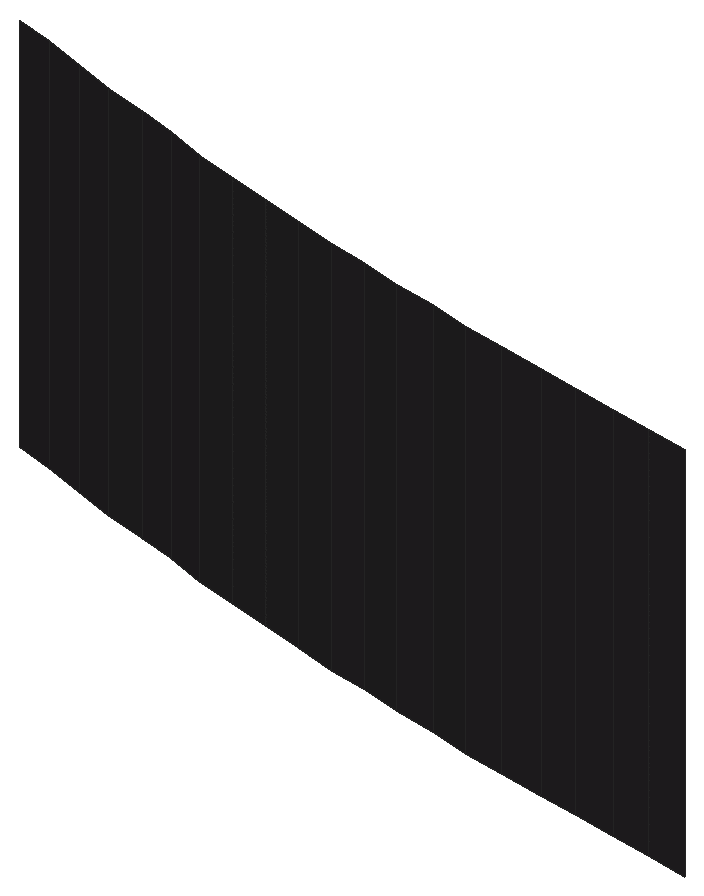
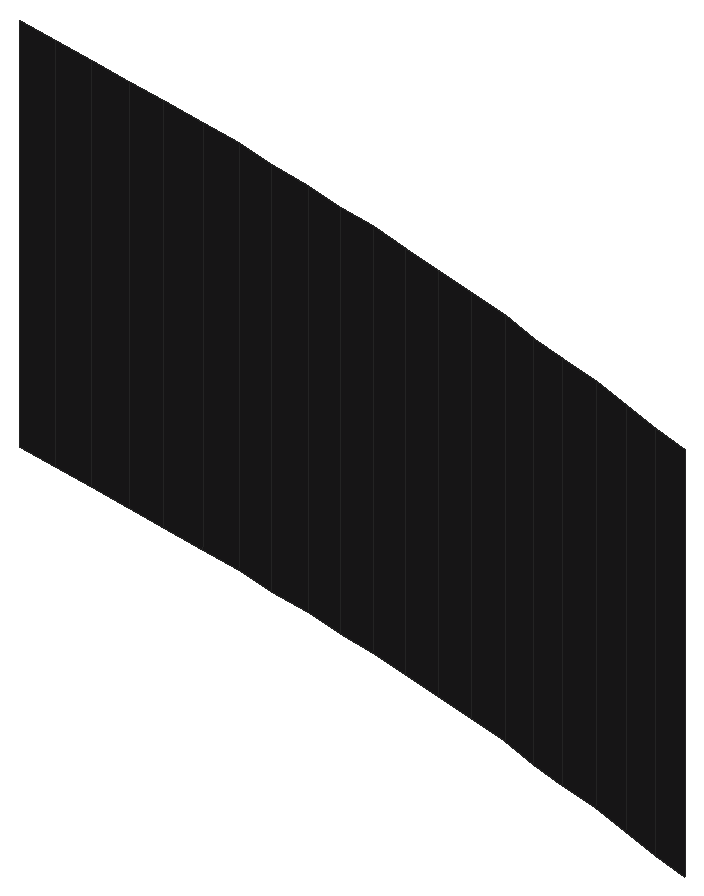
# SketchUp Ruby script. Lengths in inches.
U = 1.inch
M = Sketchup.active_model
def pt(a) = Geom::Point3d.new(a.map { |v| v * U })
def face(e, loops, mat)
  f = e.add_face(loops[0].map { |a| pt(a) })
  loops[1..].each { |l| e.add_face(l.map { |a| pt(a) }).erase! }
  f.material = f.back_material = mat if mat
  f
end
# faces: each face lists its corners as indices into pts; further lists are holes
def faces(e, pts, list, mat = nil) = list.each { |f| face(e, (f[0].is_a?(Array) ? f : [f]).map { |l| l.map { |i| pts[i] } }, mat) }
# xy, xz, yz: faces in a plane at the given z, y or x. An outline is a flat list of corners, or four numbers for a rectangle; further outlines are holes
def ring(l) = l.size == 4 ? [[l[0], l[1]], [l[2], l[1]], [l[2], l[3]], [l[0], l[3]]] : l.each_slice(2).to_a
def flat(e, list, mat, &to3) = list.each { |f| face(e, (f[0].is_a?(Array) ? f : [f]).map { |l| ring(l).map { |u, v| to3.(u, v) } }, mat) }
def xy(e, z, list, mat = nil) = flat(e, list, mat) { |x, y| [x, y, z] }
def xz(e, y, list, mat = nil) = flat(e, list, mat) { |x, z| [x, y, z] }
def yz(e, x, list, mat = nil) = flat(e, list, mat) { |y, z| [x, y, z] }
def lines(e, pts, list) = list.each { |a, b| e.add_line(pt(pts[a]), pt(pts[b])) }
# prism: a flat outline (further loops are holes) pulled along v
def prism(e, loops, v, mat = nil)
  f = face(e, loops, mat); d = Geom::Vector3d.new(v.map { |x| x * U })
  f.pushpull(f.normal.samedirection?(d) ? d.length : -d.length)
end
def box(e, o, s, mat = nil) = prism(e, [[o, [o[0] + s[0], o[1], o[2]], [o[0] + s[0], o[1] + s[1], o[2]], [o[0], o[1] + s[1], o[2]]]], [0, 0, s[2]], mat)
def at(x, y, z, deg = 0) = Geom::Transformation.translation(pt([x, y, z])) * Geom::Transformation.rotation(ORIGIN, Z_AXIS, deg.degrees)
def axes(o, x, y, z) = Geom::Transformation.new([*x, 0, *y, 0, *z, 0, *pt(o).to_a, 1])
def part(name) = M.definitions.add(name)
# library, detail: a bought-in or finely detailed component or shape, given as its bounding box
def library(name, o, s) = part(name).tap { |d| box(d.entities, o, s) }
def detail(e, o, s) = box(e.add_group.entities, o, s)
def put(e, d, t, mat = nil) = e.add_instance(d, t).tap { |i| i.material = mat if mat }
def group(e, t, mat = nil) = e.add_group.tap { |g| g.transformation = t; g.material = mat if mat }.entities
root = M.entities
M.materials.add("Marble_07_1K").color = [36, 34, 36]
p = [[345.4375,772.77,18],[345.55,772.75,18],[345.55,772.75,19],[345.4375,772.77,19],[345.66,772.73,18],[345.66,772.73,19],
  [345.77,772.71,18],[345.77,772.71,19],[344.99,772.86,18],[345.1,772.83,18],[345.1,772.83,19],[344.99,772.86,19],
  [345.21,772.81,18],[345.21,772.81,19],[345.33,772.79,18],[345.33,772.79,19],[344.56,772.96,18],[344.67,772.93,18],
  [344.67,772.93,19],[344.56,772.96,19],[344.77,772.91,18],[344.77,772.91,19],[344.88,772.88,18],[344.88,772.88,19],
  [344.23,773.05,18],[344.34,773.02,18],[344.34,773.02,19],[344.23,773.05,19],[344.45,772.99,18],[344.45,772.99,19],
  [343.91,773.15,18],[344.02,773.12,18],[344.02,773.12,19],[343.91,773.15,19],[344.12,773.09,18],[344.12,773.09,19],
  [343.59,773.26,18],[343.69,773.23,18],[343.69,773.23,19],[343.59,773.26,19],[343.8,773.19,18],[343.8,773.19,19]]
faces(root,p,[[0,1,2,3],[1,4,5,2],[4,6,7,5],[8,9,10,11],[9,12,13,10],[12,14,15,13],[14,0,3,15],[16,17,18,19],
  [17,20,21,18],[20,22,23,21],[22,8,11,23],[24,25,26,27],[25,28,29,26],[28,16,19,29],[30,31,32,33],[31,34,35,32],
  [34,24,27,35],[36,37,38,39],[37,40,41,38],[40,30,33,41]],"Marble_07_1K")
